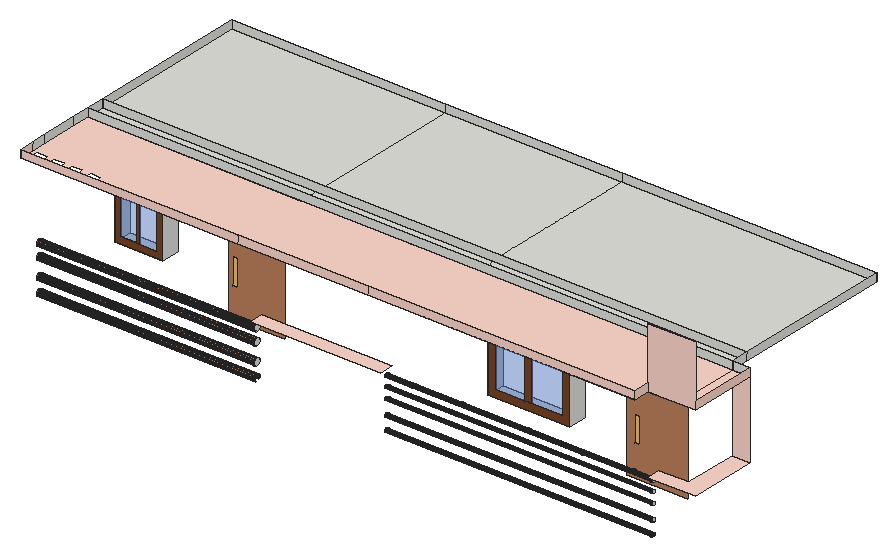
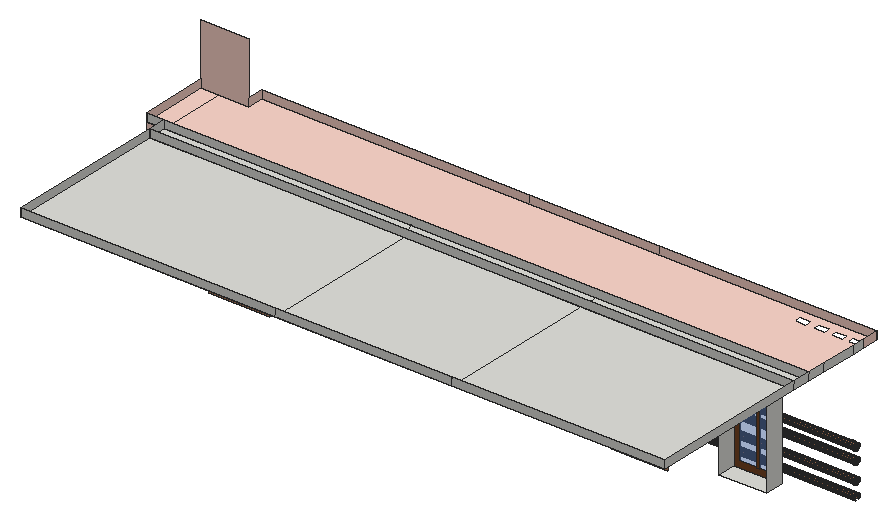
# SketchUp Ruby script. Lengths in inches.
U = 1.inch
M = Sketchup.active_model
def pt(a) = Geom::Point3d.new(a.map { |v| v * U })
def face(e, loops, mat)
  f = e.add_face(loops[0].map { |a| pt(a) })
  loops[1..].each { |l| e.add_face(l.map { |a| pt(a) }).erase! }
  f.material = f.back_material = mat if mat
  f
end
# faces: each face lists its corners as indices into pts; further lists are holes
def faces(e, pts, list, mat = nil) = list.each { |f| face(e, (f[0].is_a?(Array) ? f : [f]).map { |l| l.map { |i| pts[i] } }, mat) }
# xy, xz, yz: faces in a plane at the given z, y or x. An outline is a flat list of corners, or four numbers for a rectangle; further outlines are holes
def ring(l) = l.size == 4 ? [[l[0], l[1]], [l[2], l[1]], [l[2], l[3]], [l[0], l[3]]] : l.each_slice(2).to_a
def flat(e, list, mat, &to3) = list.each { |f| face(e, (f[0].is_a?(Array) ? f : [f]).map { |l| ring(l).map { |u, v| to3.(u, v) } }, mat) }
def xy(e, z, list, mat = nil) = flat(e, list, mat) { |x, y| [x, y, z] }
def xz(e, y, list, mat = nil) = flat(e, list, mat) { |x, z| [x, y, z] }
def yz(e, x, list, mat = nil) = flat(e, list, mat) { |y, z| [x, y, z] }
def lines(e, pts, list) = list.each { |a, b| e.add_line(pt(pts[a]), pt(pts[b])) }
# prism: a flat outline (further loops are holes) pulled along v
def prism(e, loops, v, mat = nil)
  f = face(e, loops, mat); d = Geom::Vector3d.new(v.map { |x| x * U })
  f.pushpull(f.normal.samedirection?(d) ? d.length : -d.length)
end
def box(e, o, s, mat = nil) = prism(e, [[o, [o[0] + s[0], o[1], o[2]], [o[0] + s[0], o[1] + s[1], o[2]], [o[0], o[1] + s[1], o[2]]]], [0, 0, s[2]], mat)
def at(x, y, z, deg = 0) = Geom::Transformation.translation(pt([x, y, z])) * Geom::Transformation.rotation(ORIGIN, Z_AXIS, deg.degrees)
def axes(o, x, y, z) = Geom::Transformation.new([*x, 0, *y, 0, *z, 0, *pt(o).to_a, 1])
def part(name) = M.definitions.add(name)
# library, detail: a bought-in or finely detailed component or shape, given as its bounding box
def library(name, o, s) = part(name).tap { |d| box(d.entities, o, s) }
def detail(e, o, s) = box(e.add_group.entities, o, s)
def put(e, d, t, mat = nil) = e.add_instance(d, t).tap { |i| i.material = mat if mat }
def group(e, t, mat = nil) = e.add_group.tap { |g| g.transformation = t; g.material = mat if mat }.entities
root = M.entities
M.materials.add("[Color B01]").color = [255, 216, 204]
M.materials.add("[Translucent Glass Blue]").color = [100, 149, 237]
M.materials["[Translucent Glass Blue]"].alpha = 0.5
M.materials.add("[Wood OSB]").color = [240, 195, 122]
M.materials.add("[Wood Veneer 01]1").color = [120, 70, 37]
M.materials.add("[Wood Veneer 02]").color = [190, 128, 91]
xy(root,835.8,[[1869.71,571.9,2235.65,653.97]])
xy(root,864.76,[[200.6,571.9,415.54,653.97]])
xy(root,937.9375,[[887.4375,281.88,890.53,282.28,893.41,283.48,895.88,285.375,897.77,287.85,898.97,290.73,899.375,293.82,898.97,296.91,897.77,299.78,895.88,302.26,893.41,304.15,890.53,305.35,887.4375,305.75,884.35,305.35,881.47,304.15,879,302.26,877.1,299.78,875.91,296.91,875.5,293.82,875.91,290.73,877.1,287.85,879,285.375,881.47,283.48,884.35,282.28]])
xy(root,938.37,[[681.04,286.54,699.71,286.54,700.71,287.85,701.9,290.73,702.3125,293.82,701.9,296.91,700.71,299.78,698.81,302.26,696.34,304.15,693.46,305.35,690.375,305.75,687.28,305.35,684.41,304.15,681.93,302.26,680.04,299.78,678.84,296.91,678.4375,293.82,678.84,290.73,680.04,287.85]])
xy(root,938.37,[[690.375,281.88,693.46,282.28,696.34,283.48,698.81,285.375,699.71,286.54,681.04,286.54,681.93,285.375,684.41,283.48,687.28,282.28]],"[Wood Veneer 02]")
xy(root,939.75,[[267.125,281.88,270.21,282.28,273.09,283.48,275.56,285.375,277.46,287.85,278.65,290.73,279.0625,293.82,278.65,296.91,277.46,299.78,275.56,302.26,273.09,304.15,270.21,305.35,267.125,305.75,264.03,305.35,261.16,304.15,258.68,302.26,256.79,299.78,255.59,296.91,255.1875,293.82,255.59,290.73,256.79,287.85,258.68,285.375,261.16,283.48,264.03,282.28]])
xy(root,941.3125,[[459.6875,281.88,462.78,282.28,465.66,283.48,468.13,285.375,470.02,287.85,471.22,290.73,471.625,293.82,471.22,296.91,470.02,299.78,468.13,302.26,465.66,304.15,462.78,305.35,459.6875,305.75,456.6,305.35,453.72,304.15,451.25,302.26,449.35,299.78,448.16,296.91,447.75,293.82,448.16,290.73,449.35,287.85,451.25,285.375,453.72,283.48,456.6,282.28]],"[Wood Veneer 02]")
xy(root,945.43,[[111.625,281.88,114.71,282.28,117.59,283.48,120.06,285.375,121.96,287.85,122.2,288.43,101.05,288.43,101.29,287.85,103.18,285.375,105.66,283.48,108.53,282.28],[101.05,288.43,122.2,288.43,123.15,290.73,123.5625,293.82,123.15,296.91,121.96,299.78,120.06,302.26,117.59,304.15,114.71,305.35,111.625,305.75,108.53,305.35,105.66,304.15,103.18,302.26,101.29,299.78,100.09,296.91,99.6875,293.82,100.09,290.73]])
xy(root,949.5,[[2506.15,293.09,2526,293.09,2527.76,295.4,2529.11,298.65,2529.57,302.15,2529.11,305.64,2528.66,306.73,2503.49,306.73,2503.03,305.64,2502.57,302.15,2503.03,298.65,2504.38,295.4]])
xy(root,949.5,[[2516.07,288.65,2519.57,289.11,2522.82,290.45,2525.62,292.6,2526,293.09,2506.15,293.09,2506.53,292.6,2509.32,290.45,2512.58,289.11],[2503.49,306.73,2528.66,306.73,2527.76,308.9,2525.62,311.69,2522.82,313.84,2519.57,315.1875,2516.07,315.65,2512.58,315.1875,2509.32,313.84,2506.53,311.69,2504.38,308.9]],"[Wood Veneer 02]")
xy(root,949.9375,[[1753.2,288.65,1756.69,289.11,1759.95,290.45,1762.74,292.6,1764.89,295.4,1766.24,298.65,1766.7,302.15,1766.24,305.64,1764.89,308.9,1762.74,311.69,1759.95,313.84,1756.69,315.1875,1753.2,315.65,1749.7,315.1875,1746.45,313.84,1743.65,311.69,1741.51,308.9,1740.16,305.64,1739.7,302.15,1740.16,298.65,1741.51,295.4,1743.65,292.6,1746.45,290.45,1749.7,289.11]],"[Wood Veneer 02]")
xy(root,951.33,[[2249.02,292.85,2268.5,292.85,2270.45,295.4,2271.8,298.65,2272.26,302.15,2271.8,305.64,2271.25,306.98,2246.27,306.98,2245.72,305.64,2245.26,302.15,2245.72,298.65,2247.07,295.4]])
xy(root,951.33,[[2258.76,288.65,2262.25,289.11,2265.51,290.45,2268.31,292.6,2268.5,292.85,2249.02,292.85,2249.21,292.6,2252.01,290.45,2255.27,289.11],[2246.27,306.98,2271.25,306.98,2270.45,308.9,2268.31,311.69,2265.51,313.84,2262.25,315.1875,2258.76,315.65,2255.27,315.1875,2252.01,313.84,2249.21,311.69,2247.07,308.9]],"[Wood Veneer 02]")
xy(root,952.5625,[[1968.45,288.65,1971.94,289.11,1975.2,290.45,1977.99,292.6,1980.14,295.4,1981.49,298.65,1981.95,302.15,1981.49,305.64,1980.14,308.9,1977.99,311.69,1975.2,313.84,1971.94,315.1875,1968.45,315.65,1964.95,315.1875,1961.7,313.84,1958.9,311.69,1956.76,308.9,1955.41,305.64,1954.95,302.15,1955.41,298.65,1956.76,295.4,1958.9,292.6,1961.7,290.45,1964.95,289.11]],"[Wood Veneer 02]")
xy(root,953.16,[[2720.46,293.09,2740.31,293.09,2742.08,295.4,2743.43,298.65,2743.89,302.15,2743.43,305.64,2742.97,306.73,2717.8,306.73,2717.35,305.64,2716.89,302.15,2717.35,298.65,2718.69,295.4]])
xy(root,953.16,[[2730.39,288.65,2733.88,289.11,2737.14,290.45,2739.93,292.6,2740.31,293.09,2720.46,293.09,2720.84,292.6,2723.64,290.45,2726.89,289.11],[2717.8,306.73,2742.97,306.73,2742.08,308.9,2739.93,311.69,2737.14,313.84,2733.88,315.1875,2730.39,315.65,2726.89,315.1875,2723.64,313.84,2720.84,311.69,2718.69,308.9]],"[Wood Veneer 02]")
xy(root,976.6875,[[1053.15,267.5625,1631.4,328.8],[2829.41,267.5625,3040.15,267.5625,3040.15,571.9,2962.22,571.9,2962.22,328.8,2829.41,328.8]],"[Color B01]")
xy(root,1201.73,[[1869.71,571.9,2235.65,653.97]])
xy(root,1230.86,[[670.44,571.9,998.42,653.97]])
xy(root,1240.57,[[200.6,571.9,415.54,653.97]])
xy(root,1249.8125,[[2455.03,571.9,2794.72,653.97]])
xy(root,1321.0625,[[77.93,571.9,1031.89,653.97],[1031.89,571.9,1031.89,653.97,1822.57,653.97,1857.32,571.9],[1857.32,571.9,1822.57,653.97,2962.22,653.97,2962.22,571.9],[77.93,653.97,1031.89,1377.24],[1031.89,653.97,1822.57,1377.24],
  [1822.57,653.97,2962.22,1377.24]])
xy(root,1321.0625,[[[77.93,195.0625,77.93,571.9,2962.22,571.9,2962.22,267.5625,2829.41,267.5625,2829.41,195.0625],[95.12,236.1875,148.18,267.5625],[171.43,236.1875,224.5,267.5625],[249.5,236.1875,302.56,267.5625],[333.31,236.1875,386.37,267.5625]],[2962.22,267.5625,3040.15,571.9]],"[Color B01]")
xz(root,195.0625,[[77.93,1321.0625,1053.15,1357.0625],[1053.15,1321.0625,1631.4,1357.0625],[1631.4,1321.0625,2829.41,1357.0625]],"[Color B01]")
xz(root,267.5625,[[2829.41,1321.0625,3040.15,1594.125]],"[Color B01]")
xz(root,571.9,[[77.93,1321.0625,2962.22,1357.0625],[2962.22,1321.0625,3040.15,1357.0625]])
xz(root,571.9,[[2962.22,976.6875,3040.15,1321.0625]],"[Color B01]")
xz(root,571.9,[[1902.66,868.74,2035,1168.79],[2064.96,868.74,2202.7,1168.79],[227.4375,891.6,295.54,1213.74],[313.29,891.6,388.7,1213.74]],"[Translucent Glass Blue]")
xz(root,571.9,[[729.17,873.57,751.42,991.63],[2527.49,873.57,2549.74,991.63]],"[Wood OSB]")
xz(root,571.9,[[[1869.71,835.8,2235.65,1201.73],[1902.66,868.74,2202.7,1168.79]],[[200.6,864.76,415.54,1240.57],[227.4375,891.6,388.7,1213.74]],[2035,868.74,2064.96,1168.79],[295.54,891.6,313.29,1213.74]],"[Wood Veneer 01]1")
xz(root,571.9,[[[2488.22,733.38,2761.52,1216.62],[2527.49,873.57,2549.74,991.63]],[[710.6,740.34,958.26,1190.71],[729.17,873.57,751.42,991.63]]],"[Wood Veneer 02]")
xz(root,653.97,[[77.93,1321.0625,2962.22,1357.0625]])
xz(root,1377.24,[[77.93,1321.0625,1031.89,1357.0625],[1031.89,1321.0625,1822.57,1357.0625],[1822.57,1321.0625,2962.22,1357.0625]])
yz(root,77.93,[[267.5625,1321.0625,328.8,1357.0625],[328.8,1321.0625,488.625,1357.0625],[488.625,1321.0625,571.9,1357.0625],[571.9,1321.0625,653.97,1357.0625],[653.97,1321.0625,1377.24,1357.0625]])
yz(root,77.93,[[195.0625,1321.0625,267.5625,1357.0625]],"[Color B01]")
yz(root,200.6,[[571.9,864.76,653.97,1240.57]])
yz(root,415.54,[[571.9,864.76,653.97,1240.57]])
yz(root,1053.15,[[300.66,787.68,304.32,788.16,307.72,789.57,310.65,791.82,312.89,794.74,314.3,798.15,314.79,801.8,314.3,805.46,312.89,808.87,310.65,811.79,307.72,814.04,304.32,815.45,300.66,815.93,297,815.45,293.6,814.04,290.67,811.79,288.43,808.87,287.02,805.46,286.54,801.8,287.02,798.15,288.43,794.74,290.67,791.82,293.6,789.57,297,788.16],[300.66,867.43,304.32,867.91,307.72,869.32,310.65,871.57,312.89,874.49,314.3,877.9,314.79,881.55,314.3,885.21,312.89,888.62,310.65,891.54,307.72,893.79,304.32,895.2,300.66,895.68,297,895.2,293.6,893.79,290.67,891.54,288.43,888.62,287.02,885.21,286.54,881.55,287.02,877.9,288.43,874.49,290.67,871.57,293.6,869.32,297,867.91],[300.66,924.24,304.32,924.72,307.72,926.13,310.65,928.38,312.89,931.3,314.3,934.71,314.79,938.37,314.3,942.02,312.89,945.43,310.65,948.35,307.72,950.6,304.32,952.01,300.66,952.49,297,952.01,293.6,950.6,290.67,948.35,288.43,945.43,287.02,942.02,286.54,938.37,287.02,934.71,288.43,931.3,290.67,928.38,293.6,926.13,297,924.72]])
yz(root,1869.71,[[571.9,835.8,653.97,1201.73]])
yz(root,2235.65,[[571.9,835.8,653.97,1201.73]])
yz(root,2829.41,[[299.91,784.77,301.74,785.01,303.44,785.71,304.91,786.83,306.03,788.3,306.73,790,306.98,791.83,306.73,793.66,306.03,795.36,304.91,796.82,303.44,797.94,301.74,798.65,299.91,798.89,298.09,798.65,296.38,797.94,294.92,796.82,293.8,795.36,293.09,793.66,292.85,791.83,293.09,790,293.8,788.3,294.92,786.83,296.38,785.71,298.09,785.01],[299.91,851.52,301.74,851.76,303.44,852.46,304.91,853.58,306.03,855.05,306.73,856.75,306.98,858.58,306.73,860.41,306.03,862.11,304.91,863.57,303.44,864.69,301.74,865.4,299.91,865.64,298.09,865.4,296.38,864.69,294.92,863.57,293.8,862.11,293.09,860.41,292.85,858.58,293.09,856.75,293.8,855.05,294.92,853.58,296.38,852.46,298.09,851.76],[299.91,899.83,301.74,900.07,303.44,900.77,304.91,901.9,306.03,903.36,306.73,905.0625,306.98,906.89,306.73,908.72,306.03,910.42,304.91,911.88,303.44,913.01,301.74,913.71,299.91,913.95,298.09,913.71,296.38,913.01,294.92,911.88,293.8,910.42,293.09,908.72,292.85,906.89,293.09,905.0625,293.8,903.36,294.92,901.9,296.38,900.77,298.09,900.07],[299.91,944.27,301.74,944.51,303.44,945.21,304.91,946.33,306.03,947.8,306.73,949.5,306.98,951.33,306.73,953.16,306.03,954.86,304.91,956.32,303.44,957.44,301.74,958.15,299.91,958.39,298.09,958.15,296.38,957.44,294.92,956.32,293.8,954.86,293.09,953.16,292.85,951.33,293.09,949.5,293.8,947.8,294.92,946.33,296.38,945.21,298.09,944.51]])
yz(root,2829.41,[[195.0625,1321.0625,267.5625,1357.0625]],"[Color B01]")
yz(root,2962.22,[[571.9,1321.0625,653.97,1357.0625],[653.97,1321.0625,1377.24,1357.0625]])
yz(root,3040.15,[[267.5625,1321.0625,571.9,1357.0625]],"[Color B01]")
p = [[2829.41,294.92,726.52],[2829.41,293.8,727.98],[1631.4,293.8,727.98],[1631.4,294.92,726.52],[2829.41,306.03,727.98],[2829.41,304.91,726.52],
  [1631.4,304.91,726.52],[1631.4,306.03,727.98],[1053.15,290.67,727.32],[1053.15,288.43,730.24],[77.93,288.43,730.24],[77.93,290.67,727.32],
  [1053.15,312.89,730.24],[1053.15,310.65,727.32],[77.93,310.65,727.32],[77.93,312.89,730.24],[2829.41,293.09,729.6875],[1631.4,293.09,729.6875],
  [2829.41,306.73,729.6875],[1631.4,306.73,729.6875],[2829.41,292.85,731.52],[1631.4,292.85,731.52],[2829.41,306.98,731.52],[1631.4,306.98,731.52],
  [1053.15,287.02,733.65],[77.93,287.02,733.65],[1053.15,314.3,733.65],[77.93,314.3,733.65],[2829.41,293.09,733.34],[1631.4,293.09,733.34],
  [2829.41,306.73,733.34],[1631.4,306.73,733.34],[2829.41,293.8,735.05],[1631.4,293.8,735.05],[2829.41,306.03,735.05],[1631.4,306.03,735.05],
  [1053.15,286.54,737.3],[77.93,286.54,737.3],[1053.15,314.79,737.3],[77.93,314.79,737.3],[2829.41,294.92,736.51],[1631.4,294.92,736.51],
  [2829.41,304.91,736.51],[1631.4,304.91,736.51],[2829.41,296.38,737.63],[1631.4,296.38,737.63],[2829.41,303.44,737.63],[1631.4,303.44,737.63],
  [1053.15,287.02,740.96],[77.93,287.02,740.96],[1053.15,314.3,740.96],[77.93,314.3,740.96],[2829.41,298.09,738.34],[1631.4,298.09,738.34],
  [2829.41,301.74,738.34],[1631.4,301.74,738.34],[2829.41,299.91,738.58],[1631.4,299.91,738.58],[1053.15,288.43,744.37],[77.93,288.43,744.37],
  [1053.15,312.89,744.37],[77.93,312.89,744.37],[1053.15,290.67,747.29],[77.93,290.67,747.29],[1053.15,310.65,747.29],[77.93,310.65,747.29],
  [1053.15,293.6,749.54],[77.93,293.6,749.54],[1053.15,307.72,749.54],[77.93,307.72,749.54],[1053.15,297,750.95],[77.93,297,750.95],
  [1053.15,304.32,750.95],[77.93,304.32,750.95],[1053.15,300.66,751.43],[77.93,300.66,751.43],[2829.41,299.91,784.77],[2829.41,298.09,785.01],
  [1631.4,298.09,785.01],[1631.4,299.91,784.77],[2829.41,301.74,785.01],[1631.4,301.74,785.01],[2829.41,296.38,785.71],[1631.4,296.38,785.71],
  [2829.41,303.44,785.71],[1631.4,303.44,785.71],[2829.41,294.92,786.83],[1631.4,294.92,786.83],[2829.41,304.91,786.83],[1631.4,304.91,786.83],
  [2829.41,293.8,788.3],[1631.4,293.8,788.3],[2829.41,306.03,788.3],[1631.4,306.03,788.3],[1053.15,300.66,787.68],[1053.15,297,788.16],
  [77.93,297,788.16],[77.93,300.66,787.68],[1053.15,304.32,788.16],[77.93,304.32,788.16],[1053.15,293.6,789.57],[77.93,293.6,789.57],
  [1053.15,307.72,789.57],[77.93,307.72,789.57],[2829.41,293.09,790],[1631.4,293.09,790],[2829.41,306.73,790],[1631.4,306.73,790],
  [1053.15,290.67,791.82],[77.93,290.67,791.82],[1053.15,310.65,791.82],[77.93,310.65,791.82],[2829.41,292.85,791.83],[1631.4,292.85,791.83],
  [2829.41,306.98,791.83],[1631.4,306.98,791.83],[1053.15,288.43,794.74],[77.93,288.43,794.74],[2829.41,293.09,793.66],[1631.4,293.09,793.66],
  [2829.41,306.73,793.66],[1631.4,306.73,793.66],[1053.15,312.89,794.74],[77.93,312.89,794.74],[2829.41,293.8,795.36],[1631.4,293.8,795.36],
  [2829.41,306.03,795.36],[1631.4,306.03,795.36],[1053.15,287.02,798.15],[77.93,287.02,798.15],[1053.15,314.3,798.15],[77.93,314.3,798.15],
  [2829.41,294.92,796.82],[1631.4,294.92,796.82],[2829.41,304.91,796.82],[1631.4,304.91,796.82],[2829.41,296.38,797.94],[1631.4,296.38,797.94],
  [2829.41,303.44,797.94],[1631.4,303.44,797.94],[2829.41,298.09,798.65],[1631.4,298.09,798.65],[2829.41,301.74,798.65],[1631.4,301.74,798.65],
  [1053.15,286.54,801.8],[77.93,286.54,801.8],[1053.15,314.79,801.8],[77.93,314.79,801.8],[2829.41,299.91,798.89],[1631.4,299.91,798.89],
  [1053.15,287.02,805.46],[77.93,287.02,805.46],[1053.15,314.3,805.46],[77.93,314.3,805.46],[1053.15,288.43,808.87],[77.93,288.43,808.87],
  [1053.15,312.89,808.87],[77.93,312.89,808.87],[1053.15,290.67,811.79],[77.93,290.67,811.79],[1053.15,310.65,811.79],[77.93,310.65,811.79],
  [1053.15,293.6,814.04],[77.93,293.6,814.04],[1053.15,307.72,814.04],[77.93,307.72,814.04],[1053.15,297,815.45],[77.93,297,815.45],
  [1053.15,304.32,815.45],[77.93,304.32,815.45],[1053.15,300.66,815.93],[77.93,300.66,815.93],[2829.41,299.91,851.52],[2829.41,298.09,851.76],
  [1631.4,298.09,851.76],[1631.4,299.91,851.52],[2829.41,301.74,851.76],[1631.4,301.74,851.76],[2829.41,296.38,852.46],[1631.4,296.38,852.46],
  [2829.41,303.44,852.46],[1631.4,303.44,852.46],[2829.41,294.92,853.58],[1631.4,294.92,853.58],[2829.41,304.91,853.58],[1631.4,304.91,853.58],
  [2829.41,293.8,855.05],[1631.4,293.8,855.05],[2829.41,306.03,855.05],[1631.4,306.03,855.05],[2829.41,293.09,856.75],[1631.4,293.09,856.75],
  [2829.41,306.73,856.75],[1631.4,306.73,856.75],[2829.41,292.85,858.58],[1631.4,292.85,858.58],[2829.41,306.98,858.58],[1631.4,306.98,858.58],
  [2829.41,293.09,860.41],[1631.4,293.09,860.41],[2829.41,306.73,860.41],[1631.4,306.73,860.41],[2829.41,293.8,862.11],[1631.4,293.8,862.11],
  [2829.41,306.03,862.11],[1631.4,306.03,862.11],[2829.41,294.92,863.57],[1631.4,294.92,863.57],[2829.41,304.91,863.57],[1631.4,304.91,863.57],
  [2829.41,296.38,864.69],[1631.4,296.38,864.69],[2829.41,303.44,864.69],[1631.4,303.44,864.69],[2829.41,298.09,865.4],[1631.4,298.09,865.4],
  [2829.41,301.74,865.4],[1631.4,301.74,865.4],[2829.41,299.91,865.64],[1631.4,299.91,865.64],[1053.15,300.66,867.43],[1053.15,297,867.91],
  [77.93,297,867.91],[77.93,300.66,867.43],[1053.15,304.32,867.91],[77.93,304.32,867.91],[1053.15,293.6,869.32],[77.93,293.6,869.32],
  [1053.15,307.72,869.32],[77.93,307.72,869.32],[1053.15,290.67,871.57],[77.93,290.67,871.57],[1053.15,310.65,871.57],[77.93,310.65,871.57],
  [1053.15,288.43,874.49],[77.93,288.43,874.49],[1053.15,312.89,874.49],[77.93,312.89,874.49],[1053.15,287.02,877.9],[77.93,287.02,877.9],
  [1053.15,314.3,877.9],[77.93,314.3,877.9],[1053.15,286.54,881.55],[77.93,286.54,881.55],[1053.15,314.79,881.55],[77.93,314.79,881.55],
  [1053.15,287.02,885.21],[77.93,287.02,885.21],[1053.15,314.3,885.21],[77.93,314.3,885.21],[1053.15,288.43,888.62],[77.93,288.43,888.62],
  [1053.15,312.89,888.62],[77.93,312.89,888.62],[1053.15,290.67,891.54],[77.93,290.67,891.54],[1053.15,310.65,891.54],[77.93,310.65,891.54],
  [1053.15,293.6,893.79],[77.93,293.6,893.79],[1053.15,307.72,893.79],[77.93,307.72,893.79],[1053.15,297,895.2],[77.93,297,895.2],
  [1053.15,304.32,895.2],[77.93,304.32,895.2],[1053.15,300.66,895.68],[77.93,300.66,895.68],[2829.41,299.91,899.83],[2829.41,298.09,900.07],
  [1631.4,298.09,900.07],[1631.4,299.91,899.83],[2829.41,301.74,900.07],[1631.4,301.74,900.07],[2829.41,296.38,900.77],[1631.4,296.38,900.77],
  [2829.41,303.44,900.77],[1631.4,303.44,900.77],[2829.41,294.92,901.9],[1631.4,294.92,901.9],[2829.41,304.91,901.9],[1631.4,304.91,901.9],
  [2829.41,293.8,903.36],[1631.4,293.8,903.36],[2829.41,306.03,903.36],[1631.4,306.03,903.36],[2829.41,293.09,905.0625],[1631.4,293.09,905.0625],
  [2829.41,306.73,905.0625],[1631.4,306.73,905.0625],[2829.41,292.85,906.89],[1631.4,292.85,906.89],[2829.41,306.98,906.89],[1631.4,306.98,906.89],
  [2829.41,293.09,908.72],[1631.4,293.09,908.72],[2829.41,306.73,908.72],[1631.4,306.73,908.72],[2829.41,293.8,910.42],[1631.4,293.8,910.42],
  [2829.41,306.03,910.42],[1631.4,306.03,910.42],[2829.41,294.92,911.88],[1631.4,294.92,911.88],[2829.41,304.91,911.88],[1631.4,304.91,911.88],
  [2829.41,296.38,913.01],[1631.4,296.38,913.01],[2829.41,303.44,913.01],[1631.4,303.44,913.01],[2829.41,298.09,913.71],[1631.4,298.09,913.71],
  [2829.41,301.74,913.71],[1631.4,301.74,913.71],[2829.41,299.91,913.95],[1631.4,299.91,913.95],[1053.15,300.66,924.24],[1053.15,297,924.72],
  [77.93,297,924.72],[77.93,300.66,924.24],[1053.15,304.32,924.72],[77.93,304.32,924.72],[1053.15,293.6,926.13],[77.93,293.6,926.13],
  [1053.15,307.72,926.13],[77.93,307.72,926.13],[1053.15,290.67,928.38],[77.93,290.67,928.38],[1053.15,310.65,928.38],[77.93,310.65,928.38],
  [1053.15,288.43,931.3],[77.93,288.43,931.3],[1053.15,312.89,931.3],[77.93,312.89,931.3],[1053.15,287.02,934.71],[77.93,287.02,934.71],
  [1053.15,314.3,934.71],[77.93,314.3,934.71],[1053.15,286.54,938.37],[699.71,286.54,938.37],[681.04,286.54,938.37],[77.93,286.54,938.37],
  [1053.15,314.79,938.37],[77.93,314.79,938.37],[1053.15,287.02,942.02],[77.93,287.02,942.02],[1053.15,314.3,942.02],[77.93,314.3,942.02],
  [1053.15,288.43,945.43],[122.2,288.43,945.43],[101.05,288.43,945.43],[77.93,288.43,945.43],[1053.15,312.89,945.43],[77.93,312.89,945.43],
  [2829.41,299.91,944.27],[2829.41,298.09,944.51],[1631.4,298.09,944.51],[1631.4,299.91,944.27],[2829.41,301.74,944.51],[1631.4,301.74,944.51],
  [2829.41,296.38,945.21],[1631.4,296.38,945.21],[2829.41,303.44,945.21],[1631.4,303.44,945.21],[2829.41,294.92,946.33],[1631.4,294.92,946.33],
  [2829.41,304.91,946.33],[1631.4,304.91,946.33],[1053.15,290.67,948.35],[77.93,290.67,948.35],[1053.15,310.65,948.35],[77.93,310.65,948.35],
  [2829.41,293.8,947.8],[1631.4,293.8,947.8],[2829.41,306.03,947.8],[1631.4,306.03,947.8],[2829.41,293.09,949.5],[2526,293.09,949.5],
  [2506.15,293.09,949.5],[1631.4,293.09,949.5],[2829.41,306.73,949.5],[1631.4,306.73,949.5],[2503.49,306.73,949.5],[2528.66,306.73,949.5],
  [1053.15,293.6,950.6],[77.93,293.6,950.6],[1053.15,307.72,950.6],[77.93,307.72,950.6],[2829.41,292.85,951.33],[2268.5,292.85,951.33],
  [2249.02,292.85,951.33],[1631.4,292.85,951.33],[2829.41,306.98,951.33],[1631.4,306.98,951.33],[2246.27,306.98,951.33],[2271.25,306.98,951.33],
  [1053.15,297,952.01],[77.93,297,952.01],[1053.15,304.32,952.01],[77.93,304.32,952.01],[2829.41,293.09,953.16],[2740.31,293.09,953.16],
  [2720.46,293.09,953.16],[1631.4,293.09,953.16],[2829.41,306.73,953.16],[1631.4,306.73,953.16],[2717.8,306.73,953.16],[2742.97,306.73,953.16],
  [1053.15,300.66,952.49],[77.93,300.66,952.49],[2829.41,293.8,954.86],[1631.4,293.8,954.86],[2829.41,306.03,954.86],[1631.4,306.03,954.86],
  [2829.41,294.92,956.32],[1631.4,294.92,956.32],[2829.41,304.91,956.32],[1631.4,304.91,956.32],[2829.41,296.38,957.44],[1631.4,296.38,957.44],
  [2829.41,303.44,957.44],[1631.4,303.44,957.44],[2829.41,298.09,958.15],[1631.4,298.09,958.15],[2829.41,301.74,958.15],[1631.4,301.74,958.15],
  [2829.41,299.91,958.39],[1631.4,299.91,958.39]]
faces(root,p,[[0,1,2,3],[4,5,6,7],[8,9,10,11],[12,13,14,15],[1,16,17,2],[18,4,7,19],[16,20,21,17],[22,18,19,23],
  [9,24,25,10],[26,12,15,27],[20,28,29,21],[30,22,23,31],[28,32,33,29],[34,30,31,35],[24,36,37,25],[38,26,27,39],
  [32,40,41,33],[42,34,35,43],[40,44,45,41],[46,42,43,47],[36,48,49,37],[50,38,39,51],[44,52,53,45],[54,46,47,55],
  [52,56,57,53],[56,54,55,57],[48,58,59,49],[60,50,51,61],[58,62,63,59],[64,60,61,65],[62,66,67,63],[68,64,65,69],
  [66,70,71,67],[72,68,69,73],[70,74,75,71],[74,72,73,75],[76,77,78,79],[80,76,79,81],[77,82,83,78],[84,80,81,85],
  [82,86,87,83],[88,84,85,89],[86,90,91,87],[92,88,89,93],[94,95,96,97],[98,94,97,99],[95,100,101,96],[102,98,99,103],
  [90,104,105,91],[106,92,93,107],[100,108,109,101],[110,102,103,111],[104,112,113,105],[114,106,107,115],[108,116,117,109],[112,118,119,113],
  [120,114,115,121],[122,110,111,123],[118,124,125,119],[126,120,121,127],[116,128,129,117],[130,122,123,131],[124,132,133,125],[134,126,127,135],
  [132,136,137,133],[138,134,135,139],[136,140,141,137],[142,138,139,143],[128,144,145,129],[146,130,131,147],[140,148,149,141],[148,142,143,149],
  [144,150,151,145],[152,146,147,153],[150,154,155,151],[156,152,153,157],[154,158,159,155],[160,156,157,161],[158,162,163,159],[164,160,161,165],
  [162,166,167,163],[168,164,165,169],[166,170,171,167],[170,168,169,171],[172,173,174,175],[176,172,175,177],[173,178,179,174],[180,176,177,181],
  [178,182,183,179],[184,180,181,185],[182,186,187,183],[188,184,185,189],[186,190,191,187],[192,188,189,193],[190,194,195,191],[196,192,193,197],
  [194,198,199,195],[200,196,197,201],[198,202,203,199],[204,200,201,205],[202,206,207,203],[208,204,205,209],[206,210,211,207],[212,208,209,213],
  [210,214,215,211],[216,212,213,217],[214,218,219,215],[218,216,217,219],[220,221,222,223],[224,220,223,225],[221,226,227,222],[228,224,225,229],
  [226,230,231,227],[232,228,229,233],[230,234,235,231],[236,232,233,237],[234,238,239,235],[240,236,237,241],[238,242,243,239],[244,240,241,245],
  [242,246,247,243],[248,244,245,249],[246,250,251,247],[252,248,249,253],[250,254,255,251],[256,252,253,257],[254,258,259,255],[260,256,257,261],
  [258,262,263,259],[264,260,261,265],[262,266,267,263],[266,264,265,267],[268,269,270,271],[272,268,271,273],[269,274,275,270],[276,272,273,277],
  [274,278,279,275],[280,276,277,281],[278,282,283,279],[284,280,281,285],[282,286,287,283],[288,284,285,289],[286,290,291,287],[292,288,289,293],
  [290,294,295,291],[296,292,293,297],[294,298,299,295],[300,296,297,301],[298,302,303,299],[304,300,301,305],[302,306,307,303],[308,304,305,309],
  [306,310,311,307],[312,308,309,313],[310,314,315,311],[314,312,313,315],[316,317,318,319],[320,316,319,321],[317,322,323,318],[324,320,321,325],
  [322,326,327,323],[328,324,325,329],[326,330,331,327],[332,328,329,333],[330,334,335,331],[336,332,333,337],[334,338,339,340,341,335],[342,336,337,343],
  [338,344,345,341,340,339],[346,342,343,347],[344,348,349,350,351,345],[352,346,347,353],[354,355,356,357],[358,354,357,359],[355,360,361,356],[362,358,359,363],
  [360,364,365,361],[366,362,363,367],[348,368,369,351,350,349],[370,352,353,371],[364,372,373,365],[374,366,367,375],[372,376,377,378,379,373],[380,374,375,381,382,383],
  [368,384,385,369],[386,370,371,387],[376,388,389,390,391,379,378,377],[392,380,383,382,381,393,394,395],[384,396,397,385],[398,386,387,399],[388,400,401,402,403,391,390,389],[404,392,395,394,393,405,406,407],
  [396,408,409,397],[408,398,399,409],[400,410,411,403,402,401],[412,404,407,406,405,413],[410,414,415,411],[416,412,413,417],[414,418,419,415],[420,416,417,421],
  [418,422,423,419],[424,420,421,425],[422,426,427,423],[426,424,425,427]],"[Wood Veneer 02]")
